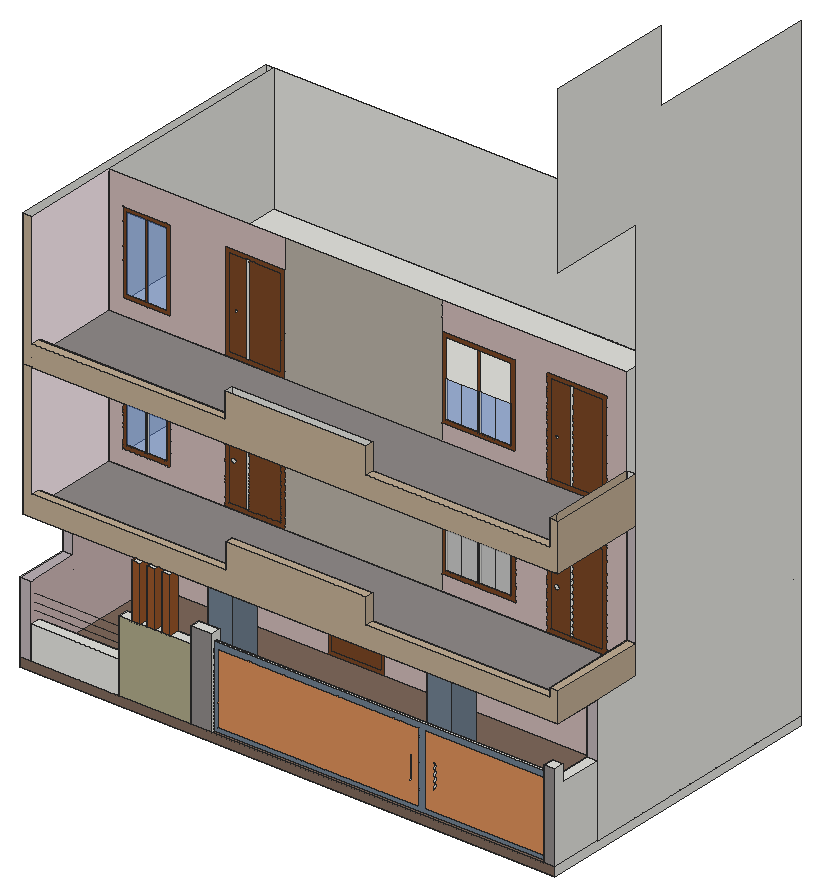
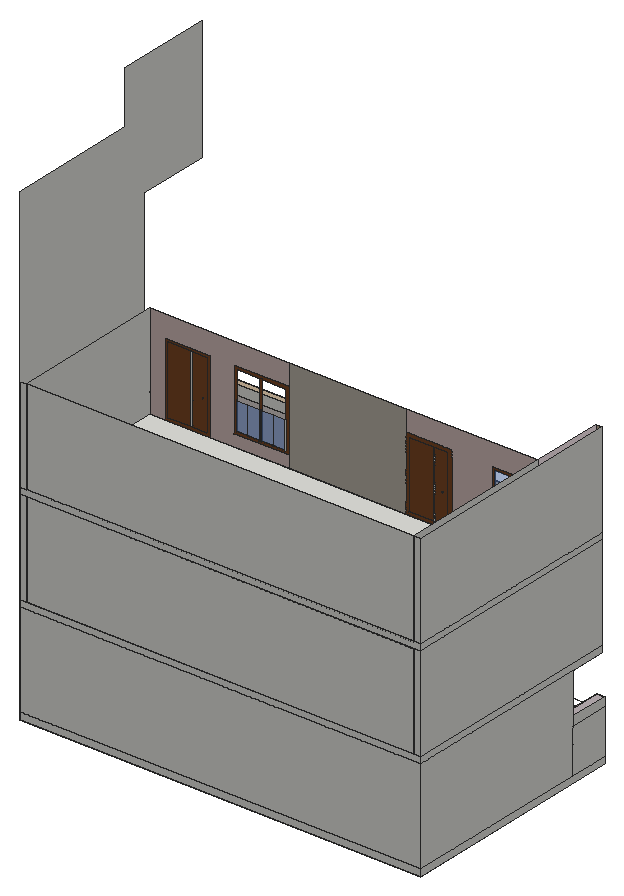
# SketchUp Ruby script. Lengths in inches.
U = 1.inch
M = Sketchup.active_model
def pt(a) = Geom::Point3d.new(a.map { |v| v * U })
def face(e, loops, mat)
  f = e.add_face(loops[0].map { |a| pt(a) })
  loops[1..].each { |l| e.add_face(l.map { |a| pt(a) }).erase! }
  f.material = f.back_material = mat if mat
  f
end
# faces: each face lists its corners as indices into pts; further lists are holes
def faces(e, pts, list, mat = nil) = list.each { |f| face(e, (f[0].is_a?(Array) ? f : [f]).map { |l| l.map { |i| pts[i] } }, mat) }
# xy, xz, yz: faces in a plane at the given z, y or x. An outline is a flat list of corners, or four numbers for a rectangle; further outlines are holes
def ring(l) = l.size == 4 ? [[l[0], l[1]], [l[2], l[1]], [l[2], l[3]], [l[0], l[3]]] : l.each_slice(2).to_a
def flat(e, list, mat, &to3) = list.each { |f| face(e, (f[0].is_a?(Array) ? f : [f]).map { |l| ring(l).map { |u, v| to3.(u, v) } }, mat) }
def xy(e, z, list, mat = nil) = flat(e, list, mat) { |x, y| [x, y, z] }
def xz(e, y, list, mat = nil) = flat(e, list, mat) { |x, z| [x, y, z] }
def yz(e, x, list, mat = nil) = flat(e, list, mat) { |y, z| [x, y, z] }
def lines(e, pts, list) = list.each { |a, b| e.add_line(pt(pts[a]), pt(pts[b])) }
# prism: a flat outline (further loops are holes) pulled along v
def prism(e, loops, v, mat = nil)
  f = face(e, loops, mat); d = Geom::Vector3d.new(v.map { |x| x * U })
  f.pushpull(f.normal.samedirection?(d) ? d.length : -d.length)
end
def box(e, o, s, mat = nil) = prism(e, [[o, [o[0] + s[0], o[1], o[2]], [o[0] + s[0], o[1] + s[1], o[2]], [o[0], o[1] + s[1], o[2]]]], [0, 0, s[2]], mat)
def at(x, y, z, deg = 0) = Geom::Transformation.translation(pt([x, y, z])) * Geom::Transformation.rotation(ORIGIN, Z_AXIS, deg.degrees)
def axes(o, x, y, z) = Geom::Transformation.new([*x, 0, *y, 0, *z, 0, *pt(o).to_a, 1])
def part(name) = M.definitions.add(name)
# library, detail: a bought-in or finely detailed component or shape, given as its bounding box
def library(name, o, s) = part(name).tap { |d| box(d.entities, o, s) }
def detail(e, o, s) = box(e.add_group.entities, o, s)
def put(e, d, t, mat = nil) = e.add_instance(d, t).tap { |i| i.material = mat if mat }
def group(e, t, mat = nil) = e.add_group.tap { |g| g.transformation = t; g.material = mat if mat }.entities
root = M.entities
M.materials.add("[0007_MistyRose]").color = [206, 184, 182]
M.materials.add("[0008_LavenderBlush]").color = [188, 177, 181]
M.materials.add("[0008_LavenderBlush]1").color = [255, 240, 245]
M.materials.add("[0012_Bisque]").color = [193, 173, 148]
M.materials.add("[0111_SlateGray]").color = [112, 128, 144]
M.materials.add("[0118_Thistle]").color = [198, 175, 198]
M.materials.add("[Beadboard]").color = [218, 143, 90]
M.materials.add("[Granite Brown]").color = [126, 104, 91]
M.materials.add("[Stone Coursed Rough]").color = [173, 168, 136]
M.materials.add("[Stone Marble]").color = [143, 138, 136]
M.materials.add("[Stone Masonry Multi]").color = [182, 175, 164]
M.materials.add("[Translucent Glass Blue]").color = [100, 149, 237]
M.materials["[Translucent Glass Blue]"].alpha = 0.5
M.materials.add("[Translucent Resin Crush Gray]").color = [184, 184, 184]
M.materials["[Translucent Resin Crush Gray]"].alpha = 0.8
M.materials.add("[Wood Cherry Original]").color = [152, 86, 42]
M.materials.add("[Wood Veneer 01]").color = [120, 70, 37]
xy(root,0,[[0,0,1524,876]])
xy(root,24,[[0,0,30,151.72],[30,0,282,30],[282,0,486,30],[486,0,546,30],[1494,0,1524,151.72],
  [0,151.72,0,876,1524,876,1524,151.72,1494,151.72,1494,849.4375,30,849.4375,30,151.72],[30,463.72,1494,849.4375]])
xy(root,24,[[546,0,1494,9.875],[546,18.16,1494,30],[[30,30,1494,439.72],[1038,151.72,1110,235.72],[414,151.72,486,235.72]]],"[Granite Brown]")
xy(root,120,[[30,0,282,30]])
xy(root,228,[[282,0,320.39,30],[320.39,0,343.01,30],[343.01,0,362.39,30],[362.39,0,385.01,30],[385.01,0,404.39,30],
  [404.39,0,427.01,30],[427.01,0,486,30],[1494,30,1524,151.72]])
xy(root,228,[[0,0,30,151.72]],"[0008_LavenderBlush]")
xy(root,252,[[546,9.875,1494,18.16]])
xy(root,274.4375,[[486,0,546,30],[1494,0,1524,30]])
xy(root,384,[[320.39,0,343.01,12],[362.39,0,385.01,12],[404.39,0,427.01,12],[[0,12,0,151.72,30,151.72,30,439.72,1494,439.72,1494,151.72,1524,151.72,1524,12,427.01,12,427.01,30,404.39,30,404.39,12,385.01,12,385.01,30,362.39,30,362.39,12,343.01,12,343.01,30,320.39,30,320.39,12],[414,151.72,486,235.72],[1038,151.72,1110,235.72]],[320.39,12,343.01,30],
  [362.39,12,385.01,30],[404.39,12,427.01,30],[30,439.72,1494,463.72],[30,463.72,1494,849.4375]])
xy(root,408,[[0,288,24,876],[24,288,1500,876]])
xy(root,408,[[24,36,1500,288]],"[Stone Marble]")
xy(root,444,[[24,12,575.91,36],[976.5625,12,1500,36]],"[0012_Bisque]")
xy(root,464.18,[[74.01,288,127.23,289],[135.23,288,188.45,289],[984.34,288,1028.68,289],[1028.68,288,1073.02,289],[1081.02,288,1125.36,289],
  [1125.36,288,1169.7,289]])
xy(root,468,[[1500,12,1524,288]],"[0012_Bisque]")
xy(root,516,[[575.91,12,976.5625,36]],"[0012_Bisque]")
xy(root,675.99,[[74.01,288,127.23,289],[135.23,288,188.45,289],[984.34,288,1028.68,289],[1028.68,288,1073.02,289],[1081.02,288,1125.36,289],
  [1125.36,288,1169.7,289]])
xy(root,768,[[0,288,24,876],[24,288,1500,876]])
xy(root,768,[[24,12,1500,288],[1500,12,1524,288]],"[0118_Thistle]")
xy(root,792,[[24,288,1500,876]])
xy(root,792,[[24,36,1500,288]],"[Stone Marble]")
xy(root,828,[[24,12,574.875,36],[976.5625,12,1500,36]],"[0012_Bisque]")
xy(root,848.18,[[984.34,288,1028.68,289],[1028.68,288,1073.02,289],[1081.02,288,1125.36,289],[1125.36,288,1169.7,289]])
xz(root,0,[[30,24,282,120]])
xz(root,0,[[0,24,30,228]],"[0008_LavenderBlush]")
xz(root,0,[[0,0,1524,24]],"[Granite Brown]")
xz(root,0,[[282,24,486,228]],"[Stone Coursed Rough]")
xz(root,0,[[486,24,546,274.4375],[1494,24,1524,274.4375]],"[Stone Marble]")
xz(root,0,[[320.39,228,343.01,384],[362.39,228,385.01,384],[404.39,228,427.01,384]],"[Wood Cherry Original]")
xz(root,9.875,[[1103.8125,93.55,1108.4375,160.18],[1171.1875,93.55,1175.8125,160.18]])
xz(root,9.875,[[[546,24,1494,252],[556.96,34.95,1129.92,236.33],[1144.77,34.95,1484.52,236.33]]],"[0111_SlateGray]")
xz(root,9.875,[[[556.96,34.95,1129.92,236.33],[1103.8125,93.55,1108.4375,160.18]],[[1144.77,34.95,1484.52,236.33],[1171.1875,93.55,1175.8125,160.18]]],"[Beadboard]")
xz(root,12,[[0,384,1524,384,1524,468,1500,468,1500,444,976.5625,444,976.5625,516,575.91,516,575.91,444,24,444,24,768,0,768],[0,768,1524,768,1524,900,1500,900,1500,828,976.5625,828,976.5625,900,574.875,900,574.875,828,24,828,24,1152,0,1152]],"[0012_Bisque]")
xz(root,18.16,[[546,24,1494,252]],"[Beadboard]")
xz(root,30,[[30,24,282,120],[282,24,486,228],[486,24,546,274.4375],[1494,228,1524,274.4375]])
xz(root,30,[[320.39,228,343.01,384],[362.39,228,385.01,384],[404.39,228,427.01,384]],"[Wood Cherry Original]")
xz(root,36,[[24,792,24,828,574.875,828,574.875,900,976.5625,900,976.5625,828,1500,828,1500,792]])
xz(root,36,[[24,408,24,444,575.91,444,575.91,516,976.5625,516,976.5625,444,1500,444,1500,408]],"[0012_Bisque]")
xz(root,151.72,[[0,228,30,384],[1494,228,1524,384]],"[0008_LavenderBlush]")
xz(root,151.72,[[414,24,486,384],[1038,24,1110,384]],"[0111_SlateGray]")
xz(root,235.72,[[414,24,486,384],[1038,24,1110,384]])
xz(root,288,[[1500,408,1524,468],[415.26,420,421.26,675.99],[1338.64,420,1344.64,675.99],[378.9,527.47,380.19,527.64,381.4,528.14,382.43,528.93,383.23,529.97,383.73,531.18,383.9,532.47,383.73,533.76,383.23,534.97,382.43,536.01,381.4,536.8,380.19,537.3,378.9,537.47,377.6,537.3,376.4,536.8,375.36,536.01,374.57,534.97,374.07,533.76,373.9,532.47,374.07,531.18,374.57,529.97,375.36,528.93,376.4,528.14,377.6,527.64],[1299.65,527.47,1300.94,527.64,1302.15,528.14,1303.18,528.93,1303.98,529.97,1304.48,531.18,1304.65,532.47,1304.48,533.76,1303.98,534.97,1303.18,536.01,1302.15,536.8,1300.94,537.3,1299.65,537.47,1298.35,537.3,1297.15,536.8,1296.11,536.01,1295.32,534.97,1294.82,533.76,1294.65,532.47,1294.82,531.18,1295.32,529.97,1296.11,528.93,1297.15,528.14,1298.35,527.64],
  [1500,792,1524,900],[415.26,804,421.26,1059.99],[1338.64,804,1344.64,1059.99]])
xz(root,288,[[[24,408,352.7,408,352.7,687.99,525.74,687.99,525.74,768,24,768],[62.01,452.18,200.45,687.99]],[972.34,408,1270.01,408,1270.01,687.99,1443.05,687.99,1443.05,408,1500,408,1500,768,972.34,768,972.34,687.99,1181.7,687.99,1181.7,452.18,972.34,452.18],[[24,792,352.7,792,352.7,1071.99,525.74,1071.99,525.74,1152,24,1152],[62.01,836.18,200.45,1071.99]],[972.34,792,1270.01,792,1270.01,1071.99,1443.05,1071.99,1443.05,792,1500,792,1500,1152,972.34,1152,972.34,1071.99,1181.7,1071.99,1181.7,836.18,972.34,836.18]],"[0007_MistyRose]")
xz(root,288,[[1500,468,1524,768]],"[0008_LavenderBlush]")
xz(root,288,[[525.74,408,972.34,768],[525.74,792,972.34,1152]],"[Stone Masonry Multi]")
xz(root,288,[[74.01,848.18,127.23,1059.99],[135.23,848.18,188.45,1059.99]],"[Translucent Glass Blue]")
xz(root,288,[[[352.7,408,525.74,687.99],[364.7,420,513.74,675.99]],[[1270.01,408,1443.05,687.99],[1282.01,420,1431.05,675.99]],[[364.7,420,415.26,675.99],[378.9,527.47,377.6,527.64,376.4,528.14,375.36,528.93,374.57,529.97,374.07,531.18,373.9,532.47,374.07,533.76,374.57,534.97,375.36,536.01,376.4,536.8,377.6,537.3,378.9,537.47,380.19,537.3,381.4,536.8,382.43,536.01,383.23,534.97,383.73,533.76,383.9,532.47,383.73,531.18,383.23,529.97,382.43,528.93,381.4,528.14,380.19,527.64]],[421.26,420,513.74,675.99],[[1282.01,420,1338.64,675.99],[1299.65,527.47,1298.35,527.64,1297.15,528.14,1296.11,528.93,1295.32,529.97,1294.82,531.18,1294.65,532.47,1294.82,533.76,1295.32,534.97,1296.11,536.01,1297.15,536.8,1298.35,537.3,1299.65,537.47,1300.94,537.3,1302.15,536.8,1303.18,536.01,1303.98,534.97,1304.48,533.76,1304.65,532.47,1304.48,531.18,1303.98,529.97,1303.18,528.93,1302.15,528.14,1300.94,527.64]],
  [1344.64,420,1431.05,675.99],[[62.01,452.18,200.45,687.99],[74.01,464.18,188.45,675.99]],[[972.34,452.18,1181.7,687.99],[984.34,464.18,1169.7,675.99]],[127.23,464.18,135.23,675.99],[1073.02,464.18,1081.02,675.99],
  [[352.7,792,525.74,1071.99],[364.7,804,513.74,1059.99]],[[1270.01,792,1443.05,1071.99],[1282.01,804,1431.05,1059.99]],[[364.7,804,415.26,1059.99],[386.84,911.22,385.54,911.39,384.34,911.89,383.3,912.68,382.51,913.72,382.01,914.93,381.84,916.22,382.01,917.51,382.51,918.72,383.3,919.76,384.34,920.55,385.54,921.05,386.84,921.22,388.13,921.05,389.34,920.55,390.37,919.76,391.17,918.72,391.67,917.51,391.84,916.22,391.67,914.93,391.17,913.72,390.37,912.68,389.34,911.89,388.13,911.39]],[421.26,804,513.74,1059.99],[[1282.01,804,1338.64,1059.99],[1299.65,911.22,1298.35,911.39,1297.15,911.89,1296.11,912.68,1295.32,913.72,1294.82,914.93,1294.65,916.22,1294.82,917.51,1295.32,918.72,1296.11,919.76,1297.15,920.55,1298.35,921.05,1299.65,921.22,1300.94,921.05,1302.15,920.55,1303.18,919.76,1303.98,918.72,1304.48,917.51,1304.65,916.22,1304.48,914.93,1303.98,913.72,1303.18,912.68,1302.15,911.89,1300.94,911.39]],
  [1344.64,804,1431.05,1059.99],[[62.01,836.18,200.45,1071.99],[74.01,848.18,188.45,1059.99]],[[972.34,836.18,1181.7,1071.99],[984.34,848.18,1169.7,1059.99]],[127.23,848.18,135.23,1059.99],[1073.02,848.18,1081.02,1059.99]],"[Wood Veneer 01]")
xz(root,289,[[74.01,464.18,127.23,675.99],[135.23,464.18,188.45,675.99],[984.34,848.18,1028.68,954.08],[1028.68,848.18,1073.02,954.08],[1081.02,848.18,1125.36,954.08],
  [1125.36,848.18,1169.7,954.08]],"[Translucent Glass Blue]")
xz(root,289,[[984.34,464.18,1028.68,570.08],[1028.68,464.18,1073.02,570.08],[1081.02,464.18,1125.36,570.08],[1125.36,464.18,1169.7,570.08],[984.34,570.08,1028.68,675.99],
  [1028.68,570.08,1073.02,675.99],[1081.02,570.08,1125.36,675.99],[1125.36,570.08,1169.7,675.99]],"[Translucent Resin Crush Gray]")
xz(root,439.72,[[[30,24,525.51,24,525.51,272.6875,687.69,272.6875,687.69,24,1494,24,1494,384,30,384],[781.14,188.9,912.81,270.27]]],"[0007_MistyRose]")
xz(root,439.72,[[793.14,200.9,846.98,229.58],[846.98,200.9,900.81,229.58],[793.14,229.58,846.98,258.27],[846.98,229.58,900.81,258.27]],"[Translucent Resin Crush Gray]")
xz(root,439.72,[[[525.51,24,687.69,272.6875],[537.51,36,675.69,260.6875]],[537.51,36,675.69,260.6875],[[781.14,188.9,912.81,270.27],[793.14,200.9,900.81,258.27]]],"[Wood Veneer 01]")
xz(root,463.72,[[30,24,1494,384]])
xz(root,849.4375,[[30,24,1494,384]])
xz(root,876,[[0,0,1524,24],[0,24,1524,384],[0,384,1524,408],[0,408,24,768],[24,408,1500,768],
  [1500,408,1524,768],[0,768,1524,792],[0,792,24,1152],[24,792,1500,1152],[1500,792,1524,1152]])
yz(root,0,[[0,0,876,24],[0,24,151.72,192],[151.72,24,876,384],[0,192,151.72,228],[12,384,876,408],
  [12,408,876,768],[12,768,876,792],[12,792,876,1152]])
yz(root,24,[[288,408,876,768],[288,792,876,1152]])
yz(root,24,[[36,408,288,408,288,768,12,768,12,444,36,444],[36,792,288,792,288,1152,12,1152,12,828,36,828]],"[0008_LavenderBlush]1")
yz(root,30,[[0,24,30,120],[439.72,24,463.72,384],[463.72,24,849.4375,384]])
yz(root,30,[[30,24,439.72,24,439.72,384,151.72,384,151.72,228,0,228,0,120,30,120]],"[0007_MistyRose]")
yz(root,74.01,[[288,464.18,289,675.99]])
yz(root,127.23,[[288,464.18,289,675.99]])
yz(root,135.23,[[288,464.18,289,675.99]])
yz(root,188.45,[[288,464.18,289,675.99]])
yz(root,282,[[0,24,30,120],[0,120,30,228]])
yz(root,320.39,[[0,228,30,384]],"[Wood Cherry Original]")
yz(root,343.01,[[0,228,30,384]],"[Wood Cherry Original]")
yz(root,362.39,[[0,228,30,384]],"[Wood Cherry Original]")
yz(root,385.01,[[0,228,30,384]],"[Wood Cherry Original]")
yz(root,404.39,[[0,228,30,384]],"[Wood Cherry Original]")
yz(root,414,[[151.72,24,235.72,384]],"[0111_SlateGray]")
yz(root,427.01,[[0,228,30,384]],"[Wood Cherry Original]")
yz(root,486,[[0,24,30,228],[0,228,30,274.4375]])
yz(root,486,[[151.72,24,235.72,384]],"[0111_SlateGray]")
yz(root,546,[[0,24,9.875,24,9.875,252,18.16,252,18.16,24,30,24,30,274.4375,0,274.4375],[9.875,24,18.16,252]])
yz(root,574.875,[[12,828,36,900]])
yz(root,575.91,[[12,444,36,516]],"[0012_Bisque]")
yz(root,976.5625,[[12,444,36,516],[12,828,36,900]],"[0012_Bisque]")
yz(root,984.34,[[288,464.18,289,570.08],[288,570.08,289,675.99],[288,848.18,289,954.08]])
yz(root,1038,[[151.72,24,235.72,384]],"[0111_SlateGray]")
yz(root,1073.02,[[288,464.18,289,570.08],[288,570.08,289,675.99],[288,848.18,289,954.08]])
yz(root,1081.02,[[288,464.18,289,570.08],[288,570.08,289,675.99],[288,848.18,289,954.08]])
yz(root,1110,[[151.72,24,235.72,384]],"[0111_SlateGray]")
yz(root,1169.7,[[288,464.18,289,570.08],[288,570.08,289,675.99],[288,848.18,289,954.08]])
yz(root,1494,[[0,24,0,274.4375,30,274.4375,30,24,18.16,24,18.16,252,9.875,252,9.875,24],[9.875,24,18.16,252],[30,24,30,228,151.72,228,151.72,384,439.72,384,439.72,24],[439.72,24,463.72,384],[463.72,24,849.4375,384]])
yz(root,1500,[[288,408,876,768],[288,792,876,1152]])
yz(root,1500,[[36,408,260.5,468],[260.5,408,288,468],[12,444,36,468],[36,792,288,900],[12,828,36,900]],"[0012_Bisque]")
yz(root,1524,[[0,0,876,24],[0,24,151.72,24,151.72,228,30,228,30,274.4375,0,274.4375],[151.72,24,876,24,876,1800,378,1800,378,2004,12,2004,12,1536,288,1536,288,384,151.72,384]])
yz(root,1524,[[12,384,288,468],[12,768,288,900]],"[0012_Bisque]")
p = [[1494,849.4375,384],[1524,849.4375,384],[24,36,792],[24,12,792],[30,151.72,192],[0,151.72,192],
  [282,15,120],[282,15,148.47],[282,15,192],[30,15,192],[282,15,169.05],[30,15,169.05],
  [30,15,148.47]]
lines(root,p,[[0,1],[2,3],[4,5],[6,7],[8,9],[10,8],[10,11],[7,10],[7,12]])
